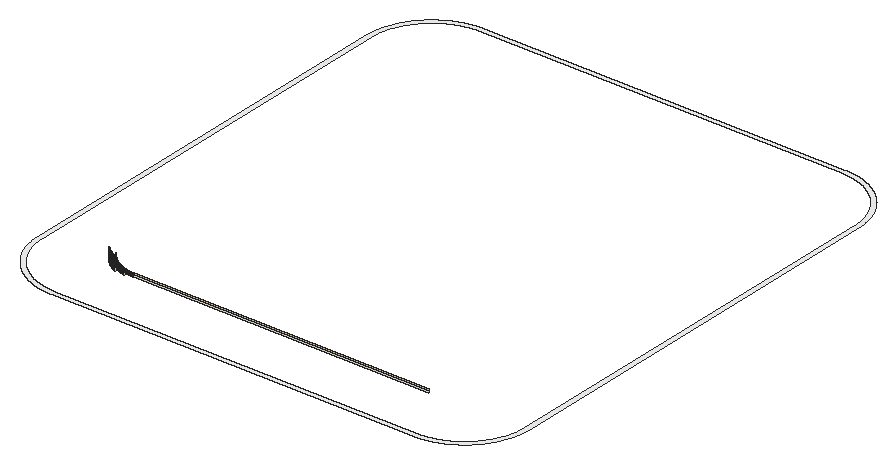
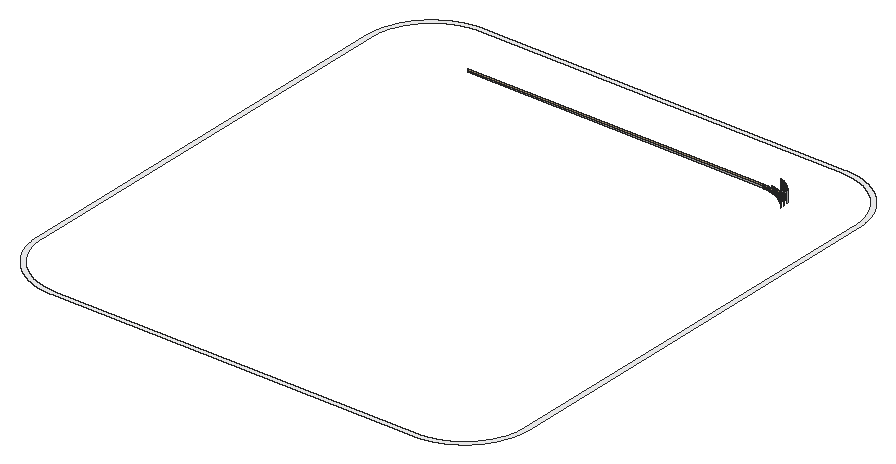
# SketchUp Ruby script. Lengths in inches.
U = 1.inch
M = Sketchup.active_model
def pt(a) = Geom::Point3d.new(a.map { |v| v * U })
def face(e, loops, mat)
  f = e.add_face(loops[0].map { |a| pt(a) })
  loops[1..].each { |l| e.add_face(l.map { |a| pt(a) }).erase! }
  f.material = f.back_material = mat if mat
  f
end
# faces: each face lists its corners as indices into pts; further lists are holes
def faces(e, pts, list, mat = nil) = list.each { |f| face(e, (f[0].is_a?(Array) ? f : [f]).map { |l| l.map { |i| pts[i] } }, mat) }
# xy, xz, yz: faces in a plane at the given z, y or x. An outline is a flat list of corners, or four numbers for a rectangle; further outlines are holes
def ring(l) = l.size == 4 ? [[l[0], l[1]], [l[2], l[1]], [l[2], l[3]], [l[0], l[3]]] : l.each_slice(2).to_a
def flat(e, list, mat, &to3) = list.each { |f| face(e, (f[0].is_a?(Array) ? f : [f]).map { |l| ring(l).map { |u, v| to3.(u, v) } }, mat) }
def xy(e, z, list, mat = nil) = flat(e, list, mat) { |x, y| [x, y, z] }
def xz(e, y, list, mat = nil) = flat(e, list, mat) { |x, z| [x, y, z] }
def yz(e, x, list, mat = nil) = flat(e, list, mat) { |y, z| [x, y, z] }
def lines(e, pts, list) = list.each { |a, b| e.add_line(pt(pts[a]), pt(pts[b])) }
# prism: a flat outline (further loops are holes) pulled along v
def prism(e, loops, v, mat = nil)
  f = face(e, loops, mat); d = Geom::Vector3d.new(v.map { |x| x * U })
  f.pushpull(f.normal.samedirection?(d) ? d.length : -d.length)
end
def box(e, o, s, mat = nil) = prism(e, [[o, [o[0] + s[0], o[1], o[2]], [o[0] + s[0], o[1] + s[1], o[2]], [o[0], o[1] + s[1], o[2]]]], [0, 0, s[2]], mat)
def at(x, y, z, deg = 0) = Geom::Transformation.translation(pt([x, y, z])) * Geom::Transformation.rotation(ORIGIN, Z_AXIS, deg.degrees)
def axes(o, x, y, z) = Geom::Transformation.new([*x, 0, *y, 0, *z, 0, *pt(o).to_a, 1])
def part(name) = M.definitions.add(name)
# library, detail: a bought-in or finely detailed component or shape, given as its bounding box
def library(name, o, s) = part(name).tap { |d| box(d.entities, o, s) }
def detail(e, o, s) = box(e.add_group.entities, o, s)
def put(e, d, t, mat = nil) = e.add_instance(d, t).tap { |i| i.material = mat if mat }
def group(e, t, mat = nil) = e.add_group.tap { |g| g.transformation = t; g.material = mat if mat }.entities
root = M.entities
M.materials.add("False Ceiling Light").color = [254, 223, 179]
M.materials.add("[Quartz Light Grey]").color = [251, 251, 252]
xy(root,115.32,[[[44.75,42,177.25,42,177.5,42.01,177.75,42.01,178.01,42.02,178.26,42.03,178.51,42.05,178.76,42.0625,179.01,42.08,179.26,42.11,179.51,42.13,179.76,42.16,180.01,42.1875,180.26,42.22,180.51,42.26,180.75,42.3,181.25,42.38,181.5,42.43,181.74,42.47,181.99,42.52,182.24,42.58,182.48,42.63,182.72,42.69,182.97,42.75,183.21,42.82,183.45,42.88,183.7,42.95,183.9375,43.02,184.18,43.1,184.42,43.17,184.66,43.25,184.89,43.33,185.37,43.51,185.6,43.59,185.83,43.69,186.07,43.78,186.53,43.97,186.76,44.07,186.99,44.18,187.22,44.28,187.45,44.39,187.67,44.5,187.9,44.62,188.12,44.73,188.34,44.85,188.5625,44.97,188.78,45.09,189,45.22,189.22,45.34,189.43,45.47,189.65,45.6,189.86,45.74,190.07,45.87,190.7,46.29,190.9,46.4375,191.11,46.58,191.51,46.88,191.71,47.04,191.91,47.19,192.1,47.35,192.3,47.51,192.68,47.83,192.87,48,193.06,48.16,193.25,48.33,193.43,48.5,193.61,48.68,193.79,48.85,194.15,49.21,194.32,49.39,194.5,49.57,194.67,49.75,194.84,49.94,195,50.13,195.17,50.32,195.49,50.7,195.65,50.9,195.81,51.09,195.96,51.29,196.12,51.49,196.42,51.89,196.5625,52.1,196.71,52.3,197.13,52.93,197.26,53.14,197.4,53.35,197.53,53.57,197.66,53.78,197.78,54,197.91,54.22,198.03,54.4375,198.15,54.66,198.27,54.88,198.38,55.1,198.5,55.33,198.61,55.55,198.72,55.78,198.82,56.01,198.93,56.24,199.03,56.47,199.22,56.93,199.31,57.17,199.41,57.4,199.49,57.63,199.67,58.11,199.75,58.34,199.83,58.58,199.9,58.82,199.98,59.0625,200.05,59.3,200.12,59.55,200.18,59.79,200.25,60.03,200.31,60.28,200.37,60.52,200.42,60.76,200.48,61.01,200.53,61.26,200.57,61.5,200.62,61.75,200.7,62.25,200.74,62.49,200.78,62.74,200.8125,62.99,200.84,63.24,200.87,63.49,200.89,63.74,200.92,63.99,200.9375,64.24,200.95,64.49,200.97,64.74,200.98,64.99,200.99,65.25,200.99,65.5,201,65.75,201,216.25,200.99,216.5,200.99,216.75,200.98,217.01,200.97,217.26,200.95,217.51,200.9375,217.76,200.92,218.01,200.89,218.26,200.87,218.51,200.84,218.76,200.8125,219.01,200.78,219.26,200.74,219.51,200.7,219.75,200.62,220.25,200.57,220.5,200.53,220.74,200.48,220.99,200.42,221.24,200.37,221.48,200.31,221.72,200.25,221.97,200.18,222.21,200.12,222.45,200.05,222.7,199.98,222.9375,199.9,223.18,199.83,223.42,199.75,223.66,199.67,223.89,199.49,224.37,199.41,224.6,199.31,224.83,199.22,225.07,199.03,225.53,198.93,225.76,198.82,225.99,198.72,226.22,198.61,226.45,198.5,226.67,198.38,226.9,198.27,227.12,198.15,227.34,198.03,227.5625,197.91,227.78,197.78,228,197.66,228.22,197.53,228.43,197.4,228.65,197.26,228.86,197.13,229.07,196.71,229.7,196.5625,229.9,196.42,230.11,196.12,230.51,195.96,230.71,195.81,230.91,195.65,231.1,195.49,231.3,195.17,231.68,195,231.87,194.84,232.06,194.67,232.25,194.5,232.43,194.32,232.61,194.15,232.79,193.79,233.15,193.61,233.32,193.43,233.5,193.25,233.67,193.06,233.84,192.87,234,192.68,234.17,192.3,234.49,192.1,234.65,191.91,234.81,191.71,234.96,191.51,235.12,191.11,235.42,190.9,235.5625,190.7,235.71,190.07,236.13,189.86,236.26,189.65,236.4,189.43,236.53,189.22,236.66,189,236.78,188.78,236.91,188.5625,237.03,188.34,237.15,188.12,237.27,187.9,237.38,187.67,237.5,187.45,237.61,187.22,237.72,186.99,237.82,186.76,237.93,186.53,238.03,186.07,238.22,185.83,238.31,185.6,238.41,185.37,238.49,184.89,238.67,184.66,238.75,184.42,238.83,184.18,238.9,183.9375,238.98,183.7,239.05,183.45,239.12,183.21,239.18,182.97,239.25,182.72,239.31,182.48,239.37,182.24,239.42,181.99,239.48,181.74,239.53,181.5,239.57,181.25,239.62,180.75,239.7,180.51,239.74,180.26,239.78,180.01,239.8125,179.76,239.84,179.51,239.87,179.26,239.89,179.01,239.92,178.76,239.9375,178.51,239.95,178.26,239.97,178.01,239.98,177.75,239.99,177.5,239.99,177.25,240,44.75,240,44.5,239.99,44.25,239.99,43.99,239.98,43.74,239.97,43.49,239.95,43.24,239.9375,42.99,239.92,42.74,239.89,42.49,239.87,42.24,239.84,41.99,239.8125,41.74,239.78,41.49,239.74,41.25,239.7,40.75,239.62,40.5,239.57,40.26,239.53,40.01,239.48,39.76,239.42,39.52,239.37,39.28,239.31,39.03,239.25,38.79,239.18,38.55,239.12,38.3,239.05,38.0625,238.98,37.82,238.9,37.58,238.83,37.34,238.75,37.11,238.67,36.63,238.49,36.4,238.41,36.17,238.31,35.93,238.22,35.47,238.03,35.24,237.93,35.01,237.82,34.78,237.72,34.55,237.61,34.33,237.5,34.1,237.38,33.88,237.27,33.66,237.15,33.4375,237.03,33.22,236.91,33,236.78,32.78,236.66,32.57,236.53,32.35,236.4,32.14,236.26,31.93,236.13,31.3,235.71,31.1,235.5625,30.89,235.42,30.49,235.12,30.29,234.96,30.09,234.81,29.9,234.65,29.7,234.49,29.32,234.17,29.13,234,28.94,233.84,28.75,233.67,28.57,233.5,28.39,233.32,28.21,233.15,27.85,232.79,27.68,232.61,27.5,232.43,27.33,232.25,27.16,232.06,27,231.87,26.83,231.68,26.51,231.3,26.35,231.1,26.19,230.91,26.04,230.71,25.88,230.51,25.58,230.11,25.4375,229.9,25.29,229.7,24.87,229.07,24.74,228.86,24.6,228.65,24.47,228.43,24.34,228.22,24.22,228,24.09,227.78,23.97,227.5625,23.85,227.34,23.73,227.12,23.62,226.9,23.5,226.67,23.39,226.45,23.28,226.22,23.18,225.99,23.07,225.76,22.97,225.53,22.78,225.07,22.69,224.83,22.59,224.6,22.51,224.37,22.33,223.89,22.25,223.66,22.17,223.42,22.1,223.18,22.02,222.9375,21.95,222.7,21.88,222.45,21.82,222.21,21.75,221.97,21.69,221.72,21.63,221.48,21.58,221.24,21.52,220.99,21.47,220.74,21.43,220.5,21.38,220.25,21.3,219.75,21.26,219.51,21.22,219.26,21.1875,219.01,21.16,218.76,21.13,218.51,21.11,218.26,21.08,218.01,21.0625,217.76,21.05,217.51,21.03,217.26,21.02,217.01,21.01,216.75,21.01,216.5,21,216.25,21,65.75,21.01,65.5,21.01,65.25,21.02,64.99,21.03,64.74,21.05,64.49,21.0625,64.24,21.08,63.99,21.11,63.74,21.13,63.49,21.16,63.24,21.1875,62.99,21.22,62.74,21.26,62.49,21.3,62.25,21.38,61.75,21.43,61.5,21.47,61.26,21.52,61.01,21.58,60.76,21.63,60.52,21.69,60.28,21.75,60.03,21.82,59.79,21.88,59.55,21.95,59.3,22.02,59.0625,22.1,58.82,22.17,58.58,22.25,58.34,22.33,58.11,22.51,57.63,22.59,57.4,22.69,57.17,22.78,56.93,22.97,56.47,23.07,56.24,23.18,56.01,23.28,55.78,23.39,55.55,23.5,55.33,23.62,55.1,23.73,54.88,23.85,54.66,23.97,54.4375,24.09,54.22,24.22,54,24.34,53.78,24.47,53.57,24.6,53.35,24.74,53.14,24.87,52.93,25.29,52.3,25.4375,52.1,25.58,51.89,25.88,51.49,26.04,51.29,26.19,51.09,26.35,50.9,26.51,50.7,26.83,50.32,27,50.13,27.16,49.94,27.33,49.75,27.5,49.57,27.68,49.39,27.85,49.21,28.21,48.85,28.39,48.68,28.57,48.5,28.75,48.33,28.94,48.16,29.13,48,29.32,47.83,29.7,47.51,29.9,47.35,30.09,47.19,30.29,47.04,30.49,46.88,30.89,46.58,31.1,46.4375,31.3,46.29,31.93,45.87,32.14,45.74,32.35,45.6,32.57,45.47,32.78,45.34,33,45.22,33.22,45.09,33.4375,44.97,33.66,44.85,33.88,44.73,34.1,44.62,34.33,44.5,34.55,44.39,34.78,44.28,35.01,44.18,35.24,44.07,35.47,43.97,35.93,43.78,36.17,43.69,36.4,43.59,36.63,43.51,37.11,43.33,37.34,43.25,37.58,43.17,37.82,43.1,38.0625,43.02,38.3,42.95,38.55,42.88,38.79,42.82,39.03,42.75,39.28,42.69,39.52,42.63,39.76,42.58,40.01,42.52,40.26,42.47,40.5,42.43,40.75,42.38,41.25,42.3,41.49,42.26,41.74,42.22,41.99,42.1875,42.24,42.16,42.49,42.13,42.74,42.11,42.99,42.08,43.24,42.0625,43.49,42.05,43.74,42.03,43.99,42.02,44.25,42.01,44.5,42.01],[44.53,43.5,44.29,43.51,44.06,43.52,43.82,43.53,43.59,43.54,43.35,43.56,43.12,43.58,42.88,43.6,42.65,43.625,42.41,43.65,41.95,43.71,41.71,43.74,41.02,43.86,40.78,43.9,40.55,43.94,39.86,44.09,39.4,44.21,39.18,44.27,38.72,44.39,38.5,44.46,38.27,44.53,38.05,44.6,37.82,44.68,37.6,44.75,37.16,44.91,36.9375,44.99,36.72,45.08,36.28,45.26,36.0625,45.35,35.85,45.45,35.63,45.54,35.21,45.74,35,45.85,34.79,45.95,34.16,46.28,33.95,46.4,33.75,46.51,33.55,46.63,33.34,46.75,33.14,46.88,32.94,47,32.75,47.13,32.35,47.39,32.16,47.52,31.97,47.66,31.77,47.8,31.58,47.9375,31.4,48.08,31.21,48.22,31.02,48.37,30.84,48.51,30.48,48.81,30.3,48.97,30.12,49.12,29.94,49.28,29.77,49.4375,29.6,49.6,29.26,49.92,28.92,50.26,28.6,50.6,28.4375,50.77,28.28,50.94,28.12,51.12,27.97,51.3,27.81,51.48,27.51,51.84,27.37,52.02,27.22,52.21,27.08,52.4,26.9375,52.58,26.8,52.77,26.66,52.97,26.52,53.16,26.39,53.35,26.13,53.75,26,53.94,25.88,54.14,25.75,54.34,25.63,54.55,25.51,54.75,25.4,54.95,25.28,55.16,24.95,55.79,24.85,56,24.74,56.21,24.54,56.63,24.45,56.85,24.35,57.0625,24.26,57.28,24.08,57.72,23.99,57.9375,23.91,58.16,23.75,58.6,23.68,58.82,23.6,59.05,23.53,59.27,23.46,59.5,23.39,59.72,23.27,60.18,23.21,60.4,23.09,60.86,22.94,61.55,22.9,61.78,22.86,62.02,22.74,62.71,22.71,62.95,22.65,63.41,22.625,63.65,22.6,63.88,22.58,64.12,22.56,64.35,22.54,64.59,22.53,64.82,22.52,65.06,22.51,65.29,22.5,65.53,22.5,216.47,22.51,216.71,22.52,216.94,22.53,217.18,22.54,217.41,22.56,217.65,22.58,217.88,22.6,218.12,22.625,218.35,22.65,218.59,22.71,219.05,22.74,219.29,22.86,219.98,22.9,220.22,22.94,220.45,23.09,221.14,23.21,221.6,23.27,221.82,23.39,222.28,23.46,222.5,23.53,222.73,23.6,222.95,23.68,223.18,23.75,223.4,23.91,223.84,23.99,224.0625,24.08,224.28,24.26,224.72,24.35,224.9375,24.45,225.15,24.54,225.37,24.74,225.79,24.85,226,24.95,226.21,25.28,226.84,25.4,227.05,25.51,227.25,25.63,227.45,25.75,227.66,25.88,227.86,26,228.06,26.13,228.25,26.39,228.65,26.52,228.84,26.66,229.03,26.8,229.23,26.9375,229.42,27.08,229.6,27.22,229.79,27.37,229.98,27.51,230.16,27.81,230.52,27.97,230.7,28.12,230.88,28.28,231.06,28.4375,231.23,28.6,231.4,28.92,231.74,29.26,232.08,29.6,232.4,29.77,232.5625,29.94,232.72,30.12,232.88,30.3,233.03,30.48,233.19,30.84,233.49,31.02,233.63,31.21,233.78,31.4,233.92,31.58,234.0625,31.77,234.2,31.97,234.34,32.16,234.48,32.35,234.61,32.75,234.87,32.94,235,33.14,235.12,33.34,235.25,33.55,235.37,33.75,235.49,33.95,235.6,34.16,235.72,34.79,236.05,35,236.15,35.21,236.26,35.63,236.46,35.85,236.55,36.0625,236.65,36.28,236.74,36.72,236.92,36.9375,237.01,37.16,237.09,37.6,237.25,37.82,237.32,38.05,237.4,38.27,237.47,38.5,237.54,38.72,237.61,39.18,237.73,39.4,237.79,39.86,237.91,40.55,238.06,40.78,238.1,41.02,238.14,41.71,238.26,41.95,238.29,42.41,238.35,42.65,238.375,42.88,238.4,43.12,238.42,43.35,238.44,43.59,238.46,43.82,238.47,44.06,238.48,44.29,238.49,44.53,238.5,177.47,238.5,177.71,238.49,177.94,238.48,178.18,238.47,178.41,238.46,178.65,238.44,178.88,238.42,179.12,238.4,179.35,238.375,179.59,238.35,180.05,238.29,180.29,238.26,180.98,238.14,181.22,238.1,181.45,238.06,182.14,237.91,182.6,237.79,182.82,237.73,183.28,237.61,183.5,237.54,183.73,237.47,183.95,237.4,184.18,237.32,184.4,237.25,184.84,237.09,185.0625,237.01,185.28,236.92,185.72,236.74,185.9375,236.65,186.15,236.55,186.37,236.46,186.79,236.26,187,236.15,187.21,236.05,187.84,235.72,188.05,235.6,188.25,235.49,188.45,235.37,188.66,235.25,188.86,235.12,189.06,235,189.25,234.87,189.65,234.61,189.84,234.48,190.03,234.34,190.23,234.2,190.42,234.0625,190.6,233.92,190.79,233.78,190.98,233.63,191.16,233.49,191.52,233.19,191.7,233.03,191.88,232.88,192.06,232.72,192.23,232.5625,192.4,232.4,192.74,232.08,193.08,231.74,193.4,231.4,193.5625,231.23,193.72,231.06,193.88,230.88,194.03,230.7,194.19,230.52,194.49,230.16,194.63,229.98,194.78,229.79,194.92,229.6,195.0625,229.42,195.2,229.23,195.34,229.03,195.48,228.84,195.61,228.65,195.87,228.25,196,228.06,196.12,227.86,196.25,227.66,196.37,227.45,196.49,227.25,196.6,227.05,196.72,226.84,197.05,226.21,197.15,226,197.26,225.79,197.46,225.37,197.55,225.15,197.65,224.9375,197.74,224.72,197.92,224.28,198.01,224.0625,198.09,223.84,198.25,223.4,198.32,223.18,198.4,222.95,198.47,222.73,198.54,222.5,198.61,222.28,198.73,221.82,198.79,221.6,198.91,221.14,199.06,220.45,199.1,220.22,199.14,219.98,199.26,219.29,199.29,219.05,199.35,218.59,199.375,218.35,199.4,218.12,199.42,217.88,199.44,217.65,199.46,217.41,199.47,217.18,199.48,216.94,199.49,216.71,199.5,216.47,199.5,65.53,199.49,65.29,199.48,65.06,199.47,64.82,199.46,64.59,199.44,64.35,199.42,64.12,199.4,63.88,199.375,63.65,199.35,63.41,199.29,62.95,199.26,62.71,199.14,62.02,199.1,61.78,199.06,61.55,198.91,60.86,198.79,60.4,198.73,60.18,198.61,59.72,198.54,59.5,198.47,59.27,198.4,59.05,198.32,58.82,198.25,58.6,198.09,58.16,198.01,57.9375,197.92,57.72,197.74,57.28,197.65,57.0625,197.55,56.85,197.46,56.63,197.26,56.21,197.15,56,197.05,55.79,196.72,55.16,196.6,54.95,196.49,54.75,196.37,54.55,196.25,54.34,196.12,54.14,196,53.94,195.87,53.75,195.61,53.35,195.48,53.16,195.34,52.97,195.2,52.77,195.0625,52.58,194.92,52.4,194.78,52.21,194.63,52.02,194.49,51.84,194.19,51.48,194.03,51.3,193.88,51.12,193.72,50.94,193.5625,50.77,193.4,50.6,193.08,50.26,192.74,49.92,192.4,49.6,192.23,49.4375,192.06,49.28,191.88,49.12,191.7,48.97,191.52,48.81,191.16,48.51,190.98,48.37,190.79,48.22,190.6,48.08,190.42,47.9375,190.23,47.8,190.03,47.66,189.84,47.52,189.65,47.39,189.25,47.13,189.06,47,188.86,46.88,188.66,46.75,188.45,46.63,188.25,46.51,188.05,46.4,187.84,46.28,187.21,45.95,187,45.85,186.79,45.74,186.37,45.54,186.15,45.45,185.9375,45.35,185.72,45.26,185.28,45.08,185.0625,44.99,184.84,44.91,184.4,44.75,184.18,44.68,183.95,44.6,183.73,44.53,183.5,44.46,183.28,44.39,182.82,44.27,182.6,44.21,182.14,44.09,181.45,43.94,181.22,43.9,180.98,43.86,180.29,43.74,180.05,43.71,179.59,43.65,179.35,43.625,179.12,43.6,178.88,43.58,178.65,43.56,178.41,43.54,178.18,43.53,177.94,43.52,177.71,43.51,177.47,43.5]]],"[Quartz Light Grey]")
xz(root,64.5,[[56.65,115.32,56.82,116.49],[56.82,115.32,57,116.49],[57,115.32,165,116.49]],"False Ceiling Light")
xz(root,64.5,[[56.65,115.32,56.82,115.91],[56.82,115.32,57,115.91],[57,115.32,165,115.91]],"[Quartz Light Grey]")
p = [[50.68,63.85,115.32],[50.49,63.93,115.32],[50.49,63.93,120],[50.68,63.85,120],[50.86,63.77,115.32],[50.86,63.77,120],
  [53.79,63.86,115.32],[53.98,63.82,115.32],[53.98,63.82,116.49],[53.79,63.86,116.49],[54.16,63.78,115.32],[54.16,63.78,116.49],
  [50.31,64.02,115.32],[50.31,64.02,120],[53.23,64,115.32],[53.42,63.95,115.32],[53.42,63.95,116.49],[53.23,64,116.49],
  [53.6,63.9,115.32],[53.6,63.9,116.49],[50.125,64.11,115.32],[50.125,64.11,120],[52.87,64.1,115.32],[53.05,64.05,115.32],
  [53.05,64.05,116.49],[52.87,64.1,116.49],[49.94,64.2,115.32],[49.94,64.2,120],[52.6875,64.16,115.32],[52.6875,64.16,116.49],
  [49.76,64.29,115.32],[49.76,64.29,120],[52.32,64.27,115.32],[52.5,64.21,115.32],[52.5,64.21,116.49],[52.32,64.27,116.49],
  [49.58,64.39,115.32],[49.58,64.39,120],[51.97,64.4,115.32],[52.14,64.34,115.32],[52.14,64.34,116.49],[51.97,64.4,116.49],
  [49.4,64.49,115.32],[49.4,64.49,120],[51.79,64.47,115.32],[51.79,64.47,116.49],[49.23,64.59,115.32],[49.23,64.59,120],
  [51.43,64.61,115.32],[51.61,64.54,115.32],[51.61,64.54,116.49],[51.43,64.61,116.49],[55.9375,64.54,115.32],[55.76,64.56,115.32],
  [55.76,64.56,116.49],[55.9375,64.54,116.49],[55.76,64.56,115.32],[55.9375,64.54,115.32],[55.9375,64.54,115.91],[55.76,64.56,115.91],
  [56.11,64.53,115.32],[56.11,64.53,116.49],[56.11,64.53,115.32],[56.11,64.53,115.91],[56.29,64.52,115.32],[56.29,64.52,116.49],
  [56.29,64.52,115.32],[56.29,64.52,115.91],[56.47,64.51,115.32],[56.47,64.51,116.49],[56.47,64.51,115.32],[56.47,64.51,115.91],
  [56.65,64.5,115.32],[56.65,64.5,116.49],[56.65,64.5,115.32],[56.65,64.5,115.91],[49.05,64.69,115.32],[49.05,64.69,120],
  [51.26,64.69,115.32],[51.26,64.69,116.49],[55.06,64.64,115.32],[54.88,64.67,115.32],[54.88,64.67,116.49],[55.06,64.64,116.49],
  [54.88,64.67,115.32],[55.06,64.64,115.32],[55.06,64.64,115.91],[54.88,64.67,115.91],[55.23,64.62,115.32],[55.23,64.62,116.49],
  [55.23,64.62,115.32],[55.23,64.62,115.91],[55.41,64.59,115.32],[55.41,64.59,116.49],[55.41,64.59,115.32],[55.41,64.59,115.91],
  [55.58,64.57,115.32],[55.58,64.57,116.49],[55.58,64.57,115.32],[55.58,64.57,115.91],[48.88,64.8,115.32],[48.88,64.8,120],
  [51.08,64.76,115.32],[51.08,64.76,116.49],[54.53,64.73,115.32],[54.36,64.76,115.32],[54.36,64.76,116.49],[54.53,64.73,116.49],
  [54.36,64.76,115.32],[54.53,64.73,115.32],[54.53,64.73,115.91],[54.36,64.76,115.91],[54.71,64.7,115.32],[54.71,64.7,116.49],
  [54.71,64.7,115.32],[54.71,64.7,115.91],[48.7,64.91,115.32],[48.7,64.91,120],[50.74,64.92,115.32],[50.91,64.84,115.32],
  [50.91,64.84,116.49],[50.74,64.92,116.49],[54.01,64.84,115.32],[53.84,64.875,115.32],[53.84,64.875,116.49],[54.01,64.84,116.49],
  [53.84,64.875,115.32],[54.01,64.84,115.32],[54.01,64.84,115.91],[53.84,64.875,115.91],[54.18,64.8,115.32],[54.18,64.8,116.49],
  [54.18,64.8,115.32],[54.18,64.8,115.91],[48.53,65.02,115.32],[48.53,65.02,120],[50.57,65.01,115.32],[50.57,65.01,116.49],
  [53.67,64.92,115.32],[53.49,64.96,115.32],[53.49,64.96,116.49],[53.67,64.92,116.49],[53.49,64.96,115.32],[53.67,64.92,115.32],
  [53.67,64.92,115.91],[53.49,64.96,115.91],[48.36,65.13,115.32],[48.36,65.13,120],[50.4,65.09,115.32],[50.4,65.09,116.49],
  [53.32,65.01,115.32],[53.15,65.06,115.32],[53.15,65.06,116.49],[53.32,65.01,116.49],[53.15,65.06,115.32],[53.32,65.01,115.32],
  [53.32,65.01,115.91],[53.15,65.06,115.91],[48.2,65.24,115.32],[48.2,65.24,120],[50.23,65.18,115.32],[50.23,65.18,116.49],
  [52.98,65.11,115.32],[52.81,65.17,115.32],[52.81,65.17,116.49],[52.98,65.11,116.49],[52.81,65.17,115.32],[52.98,65.11,115.32],
  [52.98,65.11,115.91],[52.81,65.17,115.91],[48.03,65.36,115.32],[48.03,65.36,120],[50.06,65.27,115.32],[50.06,65.27,116.49],
  [52.65,65.22,115.32],[52.48,65.28,115.32],[52.48,65.28,116.49],[52.65,65.22,116.49],[52.48,65.28,115.32],[52.65,65.22,115.32],
  [52.65,65.22,115.91],[52.48,65.28,115.91],[49.89,65.36,115.32],[49.89,65.36,116.49],[52.3125,65.34,115.32],[52.15,65.4,115.32],
  [52.15,65.4,116.49],[52.3125,65.34,116.49],[52.15,65.4,115.32],[52.3125,65.34,115.32],[52.3125,65.34,115.91],[52.15,65.4,115.91],
  [47.86,65.48,115.32],[47.86,65.48,120],[49.73,65.46,115.32],[49.73,65.46,116.49],[51.98,65.47,115.32],[51.98,65.47,116.49],
  [51.98,65.47,115.32],[51.98,65.47,115.91],[47.7,65.6,115.32],[47.7,65.6,120],[49.5625,65.55,115.32],[49.5625,65.55,116.49],
  [51.82,65.53,115.32],[51.65,65.6,115.32],[51.65,65.6,116.49],[51.82,65.53,116.49],[51.65,65.6,115.32],[51.82,65.53,115.32],
  [51.82,65.53,115.91],[51.65,65.6,115.91],[47.54,65.72,115.32],[47.54,65.72,120],[49.4,65.65,115.32],[49.4,65.65,116.49],
  [51.49,65.67,115.32],[51.49,65.67,116.49],[51.49,65.67,115.32],[51.49,65.67,115.91],[47.375,65.85,115.32],[47.375,65.85,120],
  [49.24,65.75,115.32],[49.24,65.75,116.49],[51.33,65.75,115.32],[51.17,65.82,115.32],[51.17,65.82,116.49],[51.33,65.75,116.49],
  [51.17,65.82,115.32],[51.33,65.75,115.32],[51.33,65.75,115.91],[51.17,65.82,115.91],[47.22,65.98,115.32],[47.22,65.98,120],
  [49.08,65.85,115.32],[49.08,65.85,116.49],[51.01,65.9,115.32],[51.01,65.9,116.49],[51.01,65.9,115.32],[51.01,65.9,115.91],
  [48.92,65.96,115.32],[48.92,65.96,116.49],[50.85,65.98,115.32],[50.85,65.98,116.49],[50.85,65.98,115.32],[50.85,65.98,115.91],
  [47.0625,66.11,115.32],[47.0625,66.11,120],[48.76,66.07,115.32],[48.76,66.07,116.49],[50.69,66.0625,115.32],[50.69,66.0625,116.49],
  [50.69,66.0625,115.32],[50.69,66.0625,115.91],[46.91,66.24,115.32],[46.91,66.24,120],[48.61,66.18,115.32],[48.61,66.18,116.49],
  [50.54,66.15,115.32],[50.38,66.23,115.32],[50.38,66.23,116.49],[50.54,66.15,116.49],[50.38,66.23,115.32],[50.54,66.15,115.32],
  [50.54,66.15,115.91],[50.38,66.23,115.91],[46.75,66.37,115.32],[46.75,66.37,120],[48.45,66.29,115.32],[48.45,66.29,116.49],
  [50.23,66.32,115.32],[50.23,66.32,116.49],[50.23,66.32,115.32],[50.23,66.32,115.91],[48.3,66.4,115.32],[48.3,66.4,116.49],
  [50.08,66.41,115.32],[50.08,66.41,116.49],[50.08,66.41,115.32],[50.08,66.41,115.91],[46.6,66.51,115.32],[46.6,66.51,120],
  [48.15,66.52,115.32],[48.15,66.52,116.49],[49.93,66.5,115.32],[49.93,66.5,116.49],[49.93,66.5,115.32],[49.93,66.5,115.91],
  [46.45,66.64,115.32],[46.45,66.64,120],[48,66.63,115.32],[48,66.63,116.49],[49.77,66.6,115.32],[49.77,66.6,116.49],
  [49.77,66.6,115.32],[49.77,66.6,115.91],[46.3,66.78,115.32],[46.3,66.78,120],[47.85,66.75,115.32],[47.85,66.75,116.49],
  [49.625,66.69,115.32],[49.625,66.69,116.49],[49.625,66.69,115.32],[49.625,66.69,115.91],[49.48,66.79,115.32],[49.48,66.79,116.49],
  [49.48,66.79,115.32],[49.48,66.79,115.91],[46.16,66.93,115.32],[46.16,66.93,120],[47.7,66.875,115.32],[47.7,66.875,116.49],
  [49.33,66.89,115.32],[49.33,66.89,116.49],[49.33,66.89,115.32],[49.33,66.89,115.91],[46.01,67.07,115.32],[46.01,67.07,120],
  [47.56,67,115.32],[47.56,67,116.49],[49.1875,66.99,115.32],[49.1875,66.99,116.49],[49.1875,66.99,115.32],[49.1875,66.99,115.91],
  [47.41,67.12,115.32],[47.41,67.12,116.49],[49.04,67.09,115.32],[49.04,67.09,116.49],[49.04,67.09,115.32],[49.04,67.09,115.91],
  [45.87,67.21,115.32],[45.87,67.21,120],[47.27,67.25,115.32],[47.27,67.25,116.49],[48.9,67.2,115.32],[48.9,67.2,116.49],
  [48.9,67.2,115.32],[48.9,67.2,115.91],[47.13,67.375,115.32],[47.13,67.375,116.49],[48.76,67.31,115.32],[48.76,67.31,116.49],
  [48.76,67.31,115.32],[48.76,67.31,115.91],[48.62,67.42,115.32],[48.62,67.42,116.49],[48.62,67.42,115.32],[48.62,67.42,115.91],
  [46.99,67.51,115.32],[46.99,67.51,116.49],[48.48,67.53,115.32],[48.48,67.53,116.49],[48.48,67.53,115.32],[48.48,67.53,115.91],
  [46.86,67.64,115.32],[46.86,67.64,116.49],[48.34,67.64,115.32],[48.34,67.64,116.49],[48.34,67.64,115.32],[48.34,67.64,115.91],
  [46.72,67.77,115.32],[46.72,67.77,116.49],[48.21,67.76,115.32],[48.21,67.76,116.49],[48.21,67.76,115.32],[48.21,67.76,115.91],
  [46.59,67.91,115.32],[46.59,67.91,116.49],[48.07,67.87,115.32],[48.07,67.87,116.49],[48.07,67.87,115.32],[48.07,67.87,115.91],
  [46.46,68.05,115.32],[46.46,68.05,116.49],[47.94,67.99,115.32],[47.94,67.99,116.49],[47.94,67.99,115.32],[47.94,67.99,115.91],
  [46.33,68.1875,115.32],[46.33,68.1875,116.49],[47.8125,68.11,115.32],[47.8125,68.11,116.49],[47.8125,68.11,115.32],[47.8125,68.11,115.91],
  [47.68,68.23,115.32],[47.68,68.23,116.49],[47.68,68.23,115.32],[47.68,68.23,115.91],[46.2,68.33,115.32],[46.2,68.33,116.49],
  [47.55,68.35,115.32],[47.55,68.35,116.49],[47.55,68.35,115.32],[47.55,68.35,115.91],[46.07,68.47,115.32],[46.07,68.47,116.49],
  [47.43,68.48,115.32],[47.43,68.48,116.49],[47.43,68.48,115.32],[47.43,68.48,115.91],[45.95,68.61,115.32],[45.95,68.61,116.49],
  [47.3,68.61,115.32],[47.3,68.61,116.49],[47.3,68.61,115.32],[47.3,68.61,115.91],[45.82,68.76,115.32],[45.82,68.76,116.49],
  [47.18,68.73,115.32],[47.18,68.73,116.49],[47.18,68.73,115.32],[47.18,68.73,115.91],[47.0625,68.86,115.32],[47.0625,68.86,116.49],
  [47.0625,68.86,115.32],[47.0625,68.86,115.91],[46.94,68.99,115.32],[46.94,68.99,116.49],[46.94,68.99,115.32],[46.94,68.99,115.91],
  [46.82,69.13,115.32],[46.82,69.13,116.49],[46.82,69.13,115.32],[46.82,69.13,115.91],[46.71,69.26,115.32],[46.71,69.26,116.49],
  [46.71,69.26,115.32],[46.71,69.26,115.91],[46.6,69.4,115.32],[46.6,69.4,116.49],[46.6,69.4,115.32],[46.6,69.4,115.91],
  [46.48,69.54,115.32],[46.48,69.54,116.49],[46.48,69.54,115.32],[46.48,69.54,115.91],[46.375,69.67,115.32],[46.375,69.67,116.49],
  [46.375,69.67,115.32],[46.375,69.67,115.91],[46.26,69.8125,115.32],[46.26,69.8125,116.49],[46.26,69.8125,115.32],[46.26,69.8125,115.91],
  [46.16,69.96,115.32],[46.16,69.96,116.49],[46.16,69.96,115.32],[46.16,69.96,115.91],[46.05,70.1,115.32],[46.05,70.1,116.49],
  [46.05,70.1,115.32],[46.05,70.1,115.91],[45.95,70.24,115.32],[45.95,70.24,116.49],[45.95,70.24,115.32],[45.95,70.24,115.91],
  [45.85,70.39,115.32],[45.85,70.39,116.49],[45.85,70.39,115.32],[45.85,70.39,115.91],[45.75,70.54,115.32],[45.75,70.54,116.49],
  [45.75,70.54,115.32],[45.75,70.54,115.91]]
faces(root,p,[[0,1,2,3],[4,0,3,5],[1,12,13,2],[12,20,21,13],[20,26,27,21],[26,30,31,27],[30,36,37,31],[36,42,43,37],
  [42,46,47,43],[56,57,58,59],[57,62,63,58],[62,66,67,63],[66,70,71,67],[70,74,75,71],[46,76,77,47],[84,85,86,87],
  [85,90,91,86],[90,94,95,91],[94,98,99,95],[98,56,59,99],[76,100,101,77],[108,109,110,111],[109,114,115,110],[114,84,87,115],
  [100,116,117,101],[126,127,128,129],[127,132,133,128],[132,108,111,133],[116,134,135,117],[142,143,144,145],[143,126,129,144],[134,146,147,135],
  [154,155,156,157],[155,142,145,156],[146,158,159,147],[166,167,168,169],[167,154,157,168],[158,170,171,159],[178,179,180,181],[179,166,169,180],
  [188,189,190,191],[189,178,181,190],[170,192,193,171],[198,188,191,199],[192,200,201,193],[208,209,210,211],[209,198,199,210],[200,212,213,201],
  [218,208,211,219],[212,220,221,213],[228,229,230,231],[229,218,219,230],[220,232,233,221],[238,228,231,239],[244,238,239,245],[232,246,247,233],
  [252,244,245,253],[246,254,255,247],[262,263,264,265],[263,252,253,264],[254,266,267,255],[272,262,265,273],[278,272,273,279],[266,280,281,267],
  [286,278,279,287],[280,288,289,281],[294,286,287,295],[288,296,297,289],[302,294,295,303],[306,302,303,307],[296,308,309,297],[314,306,307,315],
  [308,316,317,309],[322,314,315,323],[328,322,323,329],[316,330,331,317],[336,328,329,337],[342,336,337,343],[346,342,343,347],[352,346,347,353],
  [358,352,353,359],[364,358,359,365],[370,364,365,371],[376,370,371,377],[382,376,377,383],[386,382,383,387],[392,386,387,393],[398,392,393,399],
  [404,398,399,405],[410,404,405,411],[414,410,411,415],[418,414,415,419],[422,418,419,423],[426,422,423,427],[430,426,427,431],[434,430,431,435],
  [438,434,435,439],[442,438,439,443],[446,442,443,447],[450,446,447,451],[454,450,451,455],[458,454,455,459],[462,458,459,463]],"[Quartz Light Grey]")
faces(root,p,[[6,7,8,9],[7,10,11,8],[14,15,16,17],[15,18,19,16],[18,6,9,19],[22,23,24,25],[23,14,17,24],[28,22,25,29],
  [32,33,34,35],[33,28,29,34],[38,39,40,41],[39,32,35,40],[44,38,41,45],[48,49,50,51],[49,44,45,50],[52,53,54,55],
  [60,52,55,61],[64,60,61,65],[68,64,65,69],[72,68,69,73],[78,48,51,79],[80,81,82,83],[88,80,83,89],[92,88,89,93],
  [96,92,93,97],[53,96,97,54],[102,78,79,103],[104,105,106,107],[112,104,107,113],[81,112,113,82],[118,119,120,121],[119,102,103,120],
  [122,123,124,125],[130,122,125,131],[105,130,131,106],[136,118,121,137],[138,139,140,141],[123,138,141,124],[148,136,137,149],[150,151,152,153],
  [139,150,153,140],[160,148,149,161],[162,163,164,165],[151,162,165,152],[172,160,161,173],[174,175,176,177],[163,174,177,164],[182,172,173,183],
  [184,185,186,187],[175,184,187,176],[194,182,183,195],[185,196,197,186],[202,194,195,203],[204,205,206,207],[196,204,207,197],[214,202,203,215],
  [205,216,217,206],[222,214,215,223],[224,225,226,227],[216,224,227,217],[234,222,223,235],[225,236,237,226],[240,234,235,241],[236,242,243,237],
  [248,240,241,249],[242,250,251,243],[256,248,249,257],[258,259,260,261],[250,258,261,251],[268,256,257,269],[259,270,271,260],[274,268,269,275],
  [270,276,277,271],[282,274,275,283],[276,284,285,277],[290,282,283,291],[284,292,293,285],[298,290,291,299],[292,300,301,293],[300,304,305,301],
  [310,298,299,311],[304,312,313,305],[318,310,311,319],[312,320,321,313],[324,318,319,325],[320,326,327,321],[332,324,325,333],[326,334,335,327],
  [338,332,333,339],[334,340,341,335],[340,344,345,341],[348,338,339,349],[344,350,351,345],[354,348,349,355],[350,356,357,351],[360,354,355,361],
  [356,362,363,357],[366,360,361,367],[362,368,369,363],[372,366,367,373],[368,374,375,369],[378,372,373,379],[374,380,381,375],[380,384,385,381],
  [388,378,379,389],[384,390,391,385],[394,388,389,395],[390,396,397,391],[400,394,395,401],[396,402,403,397],[406,400,401,407],[402,408,409,403],
  [408,412,413,409],[412,416,417,413],[416,420,421,417],[420,424,425,421],[424,428,429,425],[428,432,433,429],[432,436,437,433],[436,440,441,437],
  [440,444,445,441],[444,448,449,445],[448,452,453,449],[452,456,457,453],[456,460,461,457]],"False Ceiling Light")
